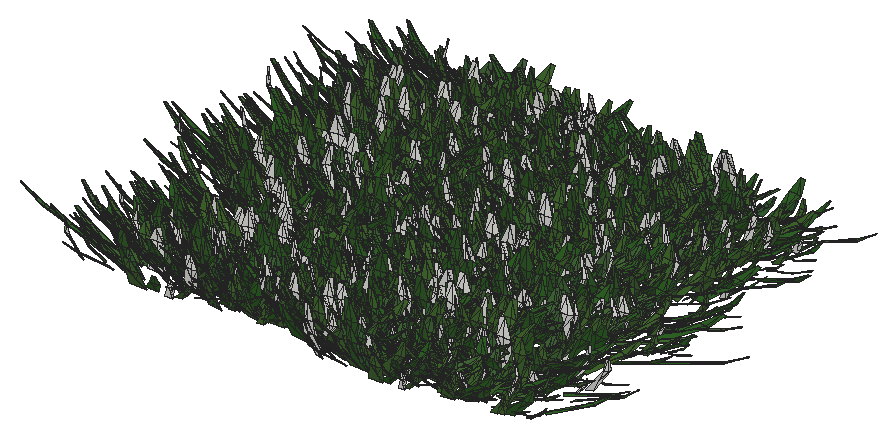
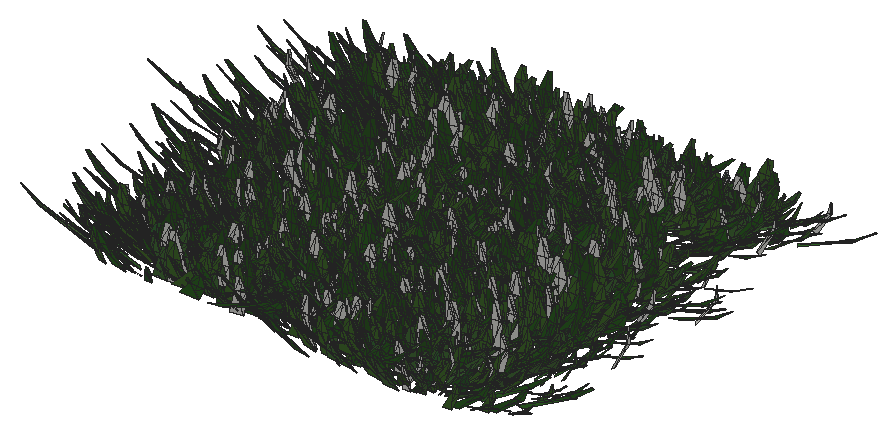
# SketchUp Ruby script. Lengths in inches.
U = 1.inch
M = Sketchup.active_model
def pt(a) = Geom::Point3d.new(a.map { |v| v * U })
def face(e, loops, mat)
  f = e.add_face(loops[0].map { |a| pt(a) })
  loops[1..].each { |l| e.add_face(l.map { |a| pt(a) }).erase! }
  f.material = f.back_material = mat if mat
  f
end
# faces: each face lists its corners as indices into pts; further lists are holes
def faces(e, pts, list, mat = nil) = list.each { |f| face(e, (f[0].is_a?(Array) ? f : [f]).map { |l| l.map { |i| pts[i] } }, mat) }
# xy, xz, yz: faces in a plane at the given z, y or x. An outline is a flat list of corners, or four numbers for a rectangle; further outlines are holes
def ring(l) = l.size == 4 ? [[l[0], l[1]], [l[2], l[1]], [l[2], l[3]], [l[0], l[3]]] : l.each_slice(2).to_a
def flat(e, list, mat, &to3) = list.each { |f| face(e, (f[0].is_a?(Array) ? f : [f]).map { |l| ring(l).map { |u, v| to3.(u, v) } }, mat) }
def xy(e, z, list, mat = nil) = flat(e, list, mat) { |x, y| [x, y, z] }
def xz(e, y, list, mat = nil) = flat(e, list, mat) { |x, z| [x, y, z] }
def yz(e, x, list, mat = nil) = flat(e, list, mat) { |y, z| [x, y, z] }
def lines(e, pts, list) = list.each { |a, b| e.add_line(pt(pts[a]), pt(pts[b])) }
# prism: a flat outline (further loops are holes) pulled along v
def prism(e, loops, v, mat = nil)
  f = face(e, loops, mat); d = Geom::Vector3d.new(v.map { |x| x * U })
  f.pushpull(f.normal.samedirection?(d) ? d.length : -d.length)
end
def box(e, o, s, mat = nil) = prism(e, [[o, [o[0] + s[0], o[1], o[2]], [o[0] + s[0], o[1] + s[1], o[2]], [o[0], o[1] + s[1], o[2]]]], [0, 0, s[2]], mat)
def at(x, y, z, deg = 0) = Geom::Transformation.translation(pt([x, y, z])) * Geom::Transformation.rotation(ORIGIN, Z_AXIS, deg.degrees)
def axes(o, x, y, z) = Geom::Transformation.new([*x, 0, *y, 0, *z, 0, *pt(o).to_a, 1])
def part(name) = M.definitions.add(name)
# library, detail: a bought-in or finely detailed component or shape, given as its bounding box
def library(name, o, s) = part(name).tap { |d| box(d.entities, o, s) }
def detail(e, o, s) = box(e.add_group.entities, o, s)
def put(e, d, t, mat = nil) = e.add_instance(d, t).tap { |i| i.material = mat if mat }
def group(e, t, mat = nil) = e.add_group.tap { |g| g.transformation = t; g.material = mat if mat }.entities
root = M.entities
M.materials.add("Material10").color = [48, 100, 38]
M.materials.add("Material3").color = [68, 110, 58]
M.materials.add("Material4").color = [48, 90, 38]
M.materials.add("Material5").color = [68, 110, 48]
M.materials.add("Material6").color = [48, 90, 48]
M.materials.add("Material7").color = [58, 110, 58]
M.materials.add("Material8").color = [58, 90, 38]
M.materials.add("Material9").color = [68, 100, 58]
c1 = part("grass00")
p = [[-0.6875,0.15,0],[-0.56,0.08,5.52],[-0.04,0.03,2.76],[0.48,-0.02,0],[0.35,-0.02,5.52],[-0.1,-0.14,5.52],
  [-0.12,0.65,8.37],[-0.42,0.65,8.37]]
faces(c1.entities,p,[[0,1,2,3],[3,2,4],[1,5,2],[5,4,2],[1,6,5],[4,5,6],[7,6,1]])
c2 = part("Group16\#1")
put(c2.entities,c1,axes([1.44,-0.61,-0.01],[0.05352,0.12609,0],[-0.10704,0.04543,0.07239],[0.06664,-0.02828,0.11628]),"Material6")
put(c2.entities,c1,axes([0.76,-0.15,-0.01],[0.04676,0.24062,0],[-0.23162,0.04501,0.06642],[0.0652,-0.01267,0.23595]),"Material3")
put(c2.entities,c1,axes([0.79,0.01,-0.01],[-0.00606,0.34651,0],[-0.34381,-0.00602,0.0432],[0.04319,0.00076,0.34386]))
put(c2.entities,c1,axes([1,0.23,-0.01],[-0.07192,0.31144,0],[-0.28722,-0.06632,0.1236],[0.12043,0.02781,0.29478]),"Material5")
put(c2.entities,c1,axes([1.66,0.77,-0.01],[-0.13828,0.29651,0],[-0.21551,-0.1005,0.22471],[0.20365,0.09498,0.23779]),"Material10")
put(c2.entities,c1,axes([0.6875,0.52,-0.01],[-0.18126,0.24051,0],[-0.22746,-0.17142,0.09788],[0.07817,0.05891,0.28481]),"Material5")
put(c2.entities,c1,axes([0.68,0.78,-0.01],[-0.215,0.18688,0],[-0.12385,-0.14248,0.21334],[0.13995,0.16101,0.18878]),"Material3")
put(c2.entities,c1,axes([0.56,1,-0.01],[-0.13756,0.07624,0],[-0.06159,-0.11112,0.0927],[0.04494,0.08108,0.12705]),"Material5")
put(c2.entities,c1,axes([0.2,0.64,-0.01],[-0.23729,0.07254,0],[-0.05711,-0.18681,0.153],[0.04473,0.14632,0.19535]),"Material10")
put(c2.entities,c1,axes([0.0625,0.72,-0.01],[-0.28874,0.02525,0],[-0.02179,-0.24916,0.14647],[0.01276,0.14591,0.25012]),"Material3")
put(c2.entities,c1,axes([-0.08,0.62,-0.01],[-0.34089,-0.04187,0],[0.03255,-0.26504,0.216],[-0.02633,0.21439,0.26703]),"Material10")
put(c2.entities,c1,axes([-0.34,0.98,-0.01],[-0.14314,-0.0493,0],[0.04397,-0.12769,0.06843],[-0.02228,0.0647,0.13505]),"Material10")
put(c2.entities,c1,axes([-0.87,1.45,-0.01],[-0.23488,-0.14114,0],[0.13761,-0.22901,0.06087],[-0.03135,0.05217,0.26717]))
put(c2.entities,c1,axes([-0.72,0.77,-0.01],[-0.14208,-0.13251,0],[0.07209,-0.0773,0.16301],[-0.11118,0.11922,0.1057]),"Material10")
put(c2.entities,c1,axes([-0.62,0.43,-0.01],[-0.14845,-0.21203,0],[0.18654,-0.13061,0.12304],[-0.10079,0.07057,0.22772]),"Material3")
put(c2.entities,c1,axes([-0.68,0.29,-0.01],[-0.13639,-0.32136,0],[0.31723,-0.13464,0.05579],[-0.05136,0.0218,0.34462]),"Material4")
put(c2.entities,c1,axes([-0.64,0.125,-0.01],[-0.0458,-0.23569,0],[0.22124,-0.043,0.08276],[-0.08124,0.01579,0.22538]),"Material7")
put(c2.entities,c1,axes([-1.6,-0.03,-0.01],[0.00576,-0.32897,0],[0.27526,0.00482,0.18018],[-0.18015,-0.00315,0.2753]),"Material5")
put(c2.entities,c1,axes([-1.36,-0.31,-0.01],[0.05718,-0.24765,0],[0.18172,0.04196,0.17267],[-0.16825,-0.03885,0.1865]),"Material10")
put(c2.entities,c1,axes([-1.54,-0.72,-0.01],[0.06537,-0.14017,0],[0.13555,0.06321,0.03939],[-0.0357,-0.01665,0.14956]))
put(c2.entities,c1,axes([-1.19,-0.9,-0.01],[0.09597,-0.12735,0],[0.11214,0.08451,0.07557],[-0.06035,-0.04548,0.14042]),"Material9")
put(c2.entities,c1,axes([-0.47,-0.54,-0.01],[0.11588,-0.10072,0],[0.0618,0.0711,0.12124],[-0.07953,-0.0915,0.0942]))
put(c2.entities,c1,axes([-0.47,-0.84,-0.01],[0.11927,-0.0661,0],[0.06603,0.11913,0.00646],[-0.00313,-0.00565,0.13621]),"Material5")
put(c2.entities,c1,axes([-0.38,-1.24,-0.01],[0.28037,-0.08571,0],[0.0618,0.20215,0.20315],[-0.05939,-0.19428,0.21139]),"Material9")
put(c2.entities,c1,axes([-0.06,-0.66,-0.01],[0.22719,-0.01987,0],[0.01247,0.14255,0.17758],[-0.01547,-0.17691,0.1431]),"Material8")
put(c2.entities,c1,axes([0.11,-0.89,-0.01],[0.14882,0.01828,0],[-0.01058,0.08611,0.12229],[0.01491,-0.12138,0.08676]),"Material6")
put(c2.entities,c1,axes([0.25,-0.72,-0.01],[0.20481,0.07053,0],[-0.06206,0.18022,0.10291],[0.03351,-0.0973,0.1906]),"Material6")
put(c2.entities,c1,axes([0.85,-1.42,-0.01],[0.16481,0.09904,0],[-0.09472,0.15762,0.05616],[0.02893,-0.04814,0.18389]),"Material5")
put(c2.entities,c1,axes([1.01,-1.09,-0.01],[0.21858,0.20385,0],[-0.17495,0.1876,0.15339],[0.10462,-0.11218,0.25652]),"Material10")
put(c2.entities,c1,axes([1.01,-0.71,-0.01],[0.08733,0.12473,0],[-0.06445,0.04512,0.13037],[0.1068,-0.07477,0.07867]),"Material6")
c3 = part("Group15\#1")
put(c3.entities,c2,at(0,0,0))
c4 = part("3darcstudiotree_grass00\#1")
put(c4.entities,c3,at(0,0,0))
put(root,c4,axes([93.18,67.32,7.6],[-0.51089,-1.13336,0],[4.16419,-0.11732,-0.02839],[0.14199,-0.004,1.31807]))
put(root,c4,axes([93.3,71.95,7.6],[-2.45945,-0.81694,0],[3.01218,-0.56677,-0.02546],[0.16778,-0.03157,1.94365]))
put(root,c4,axes([93.95,78.48,7.6],[-3.46196,-0.96436,0],[3.51371,-0.78837,-0.02493],[0.09006,-0.02021,1.43253]))
put(root,c4,axes([93.67,81.3,7.6],[-4.50327,-0.2714,0],[0.9427,-0.97764,-0.01967],[0.02949,-0.03058,1.60841]))
put(root,c4,axes([92.97,60.17,7.6],[-2.75992,0.94196,0],[-2.97534,-0.54485,-0.02032],[-0.11782,-0.02158,1.65635]))
put(root,c4,axes([93.67,46.37,7.6],[-4.30976,0.17306,0],[-0.69895,-1.08789,-0.04907],[-0.04617,-0.07186,1.63442]))
put(root,c4,axes([93.23,73.76,7.6],[1.62415,-0.82572,0],[3.47351,0.42701,-0.04022],[0.29805,0.03664,1.99791]))
put(root,c4,axes([92.31,44.43,7.6],[-0.21475,1.16093,0],[-4.31768,-0.04992,-0.00948],[-0.04784,-0.00055,1.36423]))
put(root,c4,axes([94.23,74.96,7.6],[-1.92009,-1.06648,0],[4.1428,-0.46617,-0.04331],[0.26264,-0.02955,1.88835]))
put(root,c4,axes([94.39,76.8,7.6],[-1.61898,-1.19321,0],[3.76246,-0.31906,-0.01224],[0.0924,-0.00784,1.97883]))
put(root,c4,axes([92.45,61.43,7.6],[0.9763,1.20206,0],[-4.96643,0.2521,-0.02679],[-0.14937,0.00758,1.80175]))
put(root,c4,axes([93.08,47.52,7.6],[3.61009,-0.1138,0],[0.57858,1.14719,-0.05027],[0.03392,0.06725,1.55905]))
put(root,c4,axes([92.44,70.35,7.6],[2.01763,0.79304,0],[-4.00397,0.63667,-0.00074],[-0.00407,0.00065,1.93092]))
put(root,c4,axes([94.01,55.67,7.6],[3.2052,-0.51026,0],[2.09643,0.82305,-0.0345],[0.14052,0.05517,1.8497]))
put(root,c4,axes([94.22,49.64,7.6],[0.11052,0.97112,0],[-4.47276,0.03182,-0.02239],[-0.14712,0.00105,1.83839]))
put(root,c4,axes([94.31,65.74,7.6],[-0.51157,1.00032,0],[-4.92552,-0.15743,-0.0277],[-0.16641,-0.00532,1.87956]))
put(root,c4,axes([96.53,58.84,7.6],[-2.88645,-0.88877,0],[3.86578,-0.78468,-0.02494],[0.12186,-0.02474,1.95866]))
put(root,c4,axes([96.49,82.53,7.6],[-4.37,-0.28374,0],[1.17026,-1.12647,-0.00758],[0.01125,-0.01083,1.7185]))
put(root,c4,axes([96.19,65.93,7.6],[-0.06579,-0.95839,0],[4.48291,-0.01923,-0.0405],[0.2731,-0.00117,1.89003]))
put(root,c4,axes([96.62,70.86,7.6],[-1.52084,-1.07462,0],[3.90834,-0.3457,-0.03351],[0.20602,-0.01822,1.68972]))
put(root,c4,axes([97.3,77.97,7.6],[-1.03944,-1.24074,0],[4.69727,-0.24595,-0.02019],[0.11188,-0.00586,1.69814]))
put(root,c4,axes([97.11,81.66,7.6],[-0.98612,-1.22055,0],[4.4455,-0.22448,-0.03802],[0.23503,-0.01187,1.78771]))
put(root,c4,axes([97.47,60.42,7.6],[-3.13643,-0.44743,0],[1.98712,-0.87059,-0.04344],[0.16835,-0.07376,1.9596]))
put(root,c4,axes([97.73,52.01,7.6],[-1.81933,-1.05694,0],[4.48084,-0.48206,-0.04688],[0.23644,-0.02544,1.67419]))
put(root,c4,axes([97.66,56.53,7.6],[-3.96294,0.68936,0],[-2.37942,-0.85491,-0.01001],[-0.0292,-0.01049,1.32974]))
put(root,c4,axes([98.77,64.52,7.6],[-0.37875,-1.01008,0],[4.48858,-0.10519,-0.00863],[0.04422,-0.00104,1.44957]))
put(root,c4,axes([99.4,55.39,7.6],[-1.70482,-1.13891,0],[4.74643,-0.44405,-0.05081],[0.22443,-0.021,1.49393]))
put(root,c4,axes([97.86,62.77,7.6],[4.79231,-0.42159,0],[1.43855,1.02203,-0.0057],[0.01193,0.00848,1.70987]))
put(root,c4,axes([99.49,75.21,7.6],[-0.51771,-1.03917,0],[4.88499,-0.15211,-0.06365],[0.38906,-0.01211,1.89522]))
put(root,c4,axes([99.04,72.46,7.6],[2.41645,-0.95234,0],[3.1357,0.49728,-0.01781],[0.0973,0.01543,1.50117]))
put(root,c4,axes([98.65,80.14,7.6],[3.95263,-0.39442,0],[1.50714,0.94398,-0.02611],[0.05477,0.0343,1.43783]))
put(root,c4,axes([99.95,47.45,7.6],[-4.30049,-0.11953,0],[0.50316,-1.13147,-0.05312],[0.03445,-0.07747,1.67036]))
put(root,c4,axes([98.75,46.06,7.6],[4.68959,-0.46091,0],[1.44891,0.92138,-0.00849],[0.02258,0.01436,1.79934]))
put(root,c4,axes([100.16,68.92,7.6],[0.57687,-1.07494,0],[3.69634,0.12398,-0.00096],[0.00701,0.00024,1.71349]))
put(root,c4,axes([100.13,67.55,7.6],[-4.14654,0.02565,0],[-0.12263,-1.23885,-0.01248],[-0.00137,-0.01382,1.37214]))
put(root,c4,axes([100.37,76.89,7.6],[-3.83685,0.38096,0],[-1.50034,-0.94442,-0.04199],[-0.1028,-0.06471,1.68502]))
put(root,c4,axes([100.19,61.53,7.6],[-4.14844,0.73182,0],[-2.28116,-0.8082,0],[-0.00002,-0.00001,1.91868]))
put(root,c4,axes([99.38,45.07,7.6],[3.44069,0.27197,0],[-1.2898,1.01983,-0.04459],[-0.0839,0.06634,1.66873]))
put(root,c4,axes([100.69,73.42,7.6],[-4.43528,0.66628,0],[-1.93205,-0.80382,-0.02116],[-0.06942,-0.02888,1.49339]))
put(root,c4,axes([100.37,49.59,7.6],[-2.3482,0.69512,0],[-3.39481,-0.71676,-0.03207],[-0.17565,-0.03709,1.99077]))
put(root,c4,axes([100.57,50.99,7.6],[-3.32313,0.94443,0],[-3.84247,-0.84503,-0.06393],[-0.21081,-0.04636,1.40472]))
put(root,c4,axes([100.375,53.48,7.6],[4.99296,-0.12006,0],[0.49346,1.28259,-0.06081],[0.02614,0.06795,1.44654]))
put(root,c4,axes([102.42,64.07,7.6],[-0.04021,-0.94349,0],[5.12162,-0.01364,-0.05216],[0.22205,-0.00059,1.36288]))
put(root,c4,axes([102.53,53.98,7.6],[0.15214,-1.25594,0],[4.48063,0.03392,-0.01983],[0.10676,0.00081,1.50947]))
put(root,c4,axes([102.81,76.83,7.6],[-0.76774,-1.16095,0],[4.52934,-0.18721,-0.0168],[0.08958,-0.0037,1.55067]))
put(root,c4,axes([102.96,56.75,7.6],[-4.11234,-0.7945,0],[2.93722,-0.95019,-0.06061],[0.1773,-0.05736,1.43628]))
put(root,c4,axes([102.44,65.58,7.6],[-0.59166,-1.13858,0],[3.64186,-0.11828,-0.04034],[0.25705,-0.00835,1.47504]))
put(root,c4,axes([102.7,62.67,7.6],[-3.92438,0.31948,0],[-1.16946,-0.89782,-0.04555],[-0.09619,-0.07385,1.60995]))
put(root,c4,axes([103.21,47.54,7.6],[-4.2338,0.39742,0],[-1.47473,-0.9819,-0.01194],[-0.02743,-0.01826,1.71307]))
put(root,c4,axes([103.43,52.7,7.6],[-3.93577,0.74976,0],[-2.5237,-0.82799,-0.04347],[-0.16838,-0.05524,1.66314]))
put(root,c4,axes([104.29,45.21,7.6],[-3.54943,-0.49503,0],[1.78138,-0.79829,-0.00653],[0.02016,-0.00904,1.4475]))
put(root,c4,axes([104.66,75.52,7.6],[-3.36621,-0.95264,0],[2.81846,-0.62245,-0.00245],[0.01476,-0.00326,1.8862]))
put(root,c4,axes([102.77,79.625,7.6],[0.43598,1.04612,0],[-4.32547,0.11267,-0.02993],[-0.17694,0.00461,1.61572]))
put(root,c4,axes([102.875,61.18,7.6],[-0.51235,0.89086,0],[-4.17612,-0.15011,-0.00494],[-0.0262,-0.00094,1.4129]))
put(root,c4,axes([104.84,49.36,7.6],[0.5765,-1.16396,0],[4.70538,0.14566,-0.00236],[0.01265,0.00039,1.5989]))
put(root,c4,axes([103.43,77.9,7.6],[4.23792,-0.23922,0],[0.87195,0.96546,-0.03599],[0.04234,0.04688,1.32194]))
put(root,c4,axes([104.61,67.62,7.6],[-4.26388,0.42681,0],[-1.64791,-1.02893,-0.00598],[-0.01365,-0.00852,1.70205]))
put(root,c4,axes([103.68,50.48,7.6],[4.67345,-0.08796,0],[0.29357,0.97489,-0.02417],[0.01343,0.0446,1.80918]))
put(root,c4,axes([103.74,80.78,7.6],[0.19862,1.12263,0],[-4.23211,0.0468,-0.03464],[-0.20461,0.00226,1.56527]))
put(root,c4,axes([103.5,82.27,7.6],[2.93954,0.6812,0],[-3.37406,0.90999,-0.0132],[-0.04593,0.01239,1.58767]))
put(root,c4,axes([105.44,58.21,7.6],[-4.4154,0.08876,0],[-0.37121,-1.15413,-0.04274],[-0.0155,-0.04821,1.31001]))
put(root,c4,axes([105.82,68.79,7.6],[-2.79225,-0.78906,0],[3.01148,-0.66605,-0.02762],[0.13842,-0.03061,1.68176]))
put(root,c4,axes([103.9375,59.62,7.6],[2.75191,0.75526,0],[-3.57518,0.81417,-0.05824],[-0.22433,0.05109,1.57486]))
put(root,c4,axes([105.22,71.79,7.6],[2.32702,-1.05964,0],[3.64306,0.50002,-0.02765],[0.14347,0.01969,1.53783]))
put(root,c4,axes([104.48,46.23,7.6],[2.82481,0.56439,0],[-2.40364,0.7519,-0.04441],[-0.20419,0.06387,1.772]))
put(root,c4,axes([105.49,73.35,7.6],[2.47739,-0.8352,0],[3.76427,0.69785,-0.03781],[0.14929,0.02768,1.4396]))
put(root,c4,axes([104.58,70.29,7.6],[0.70904,1.19285,0],[-3.93143,0.14606,-0.03328],[-0.20326,0.00755,1.53387]))
put(root,c4,axes([105.76,55.17,7.6],[1.81143,0.91865,0],[-4.40364,0.5427,-0.01549],[-0.06434,0.00793,1.42146]))
put(root,c4,axes([108.75,45.9,7.6],[-2.19017,-0.8406,0],[3.99666,-0.65083,-0.00487],[0.02392,-0.0039,1.74651]))
put(root,c4,axes([108.51,80.16,7.6],[-4.47501,0.4091,0],[-1.26068,-0.86189,-0.04181],[-0.08597,-0.05877,1.37365]))
put(root,c4,axes([108.81,68.65,7.6],[1.03732,-1.10415,0],[4.61468,0.27096,-0.04288],[0.24016,0.0141,1.70449]))
put(root,c4,axes([109.03,47.83,7.6],[0.84131,-0.93334,0],[4.465,0.25155,-0.02216],[0.11535,0.0065,1.52603]))
put(root,c4,axes([109.72,73.17,7.6],[-4.69083,0.06991,0],[-0.27853,-1.16812,-0.00226],[-0.00086,-0.00362,1.87745]))
put(root,c4,axes([109.36,76.69,7.6],[1.83497,-0.94895,0],[3.86157,0.46669,-0.03335],[0.17925,0.02166,1.60043]))
put(root,c4,axes([110.03,54.01,7.6],[-0.52129,-1.09873,0],[4.55576,-0.13509,-0.02638],[0.13198,-0.00391,1.44452]))
put(root,c4,axes([108.98,70.7,7.6],[4.54978,-0.41024,0],[1.68506,1.16802,-0.06016],[0.10033,0.06955,1.52593]))
put(root,c4,axes([109.26,59.98,7.6],[-1.83035,0.9083,0],[-3.79147,-0.47752,-0.03585],[-0.1914,-0.02411,1.58646]))
put(root,c4,axes([109.91,64.55,7.6],[-3.83368,0.65394,0],[-2.36906,-0.86802,-0.04776],[-0.17139,-0.0628,1.6727]))
put(root,c4,axes([109.2,58.79,7.6],[4.16884,-0.44191,0],[1.67994,0.9905,-0.02583],[0.06325,0.03729,1.68703]))
put(root,c4,axes([109.64,78.27,7.6],[5.02787,-0.3126,0],[0.9305,0.9354,-0.00031],[0.00054,0.00054,1.72722]))
put(root,c4,axes([110.24,54.98,7.6],[3.79189,-0.60703,0],[2.47223,0.9652,-0.00312],[0.00888,0.00347,1.51309]))
put(root,c4,axes([109.83,57.1,7.6],[4.87895,-0.29762,0],[0.96688,0.99066,-0.01844],[0.03122,0.03199,1.82062]))
put(root,c4,axes([110.87,72.01,7.6],[2.31216,-0.81915,0],[3.42555,0.60431,-0.01427],[0.0583,0.01029,1.30992]))
put(root,c4,axes([110.97,50.59,7.6],[2.96673,-0.89554,0],[3.5792,0.74107,-0.01649],[0.07862,0.01628,1.79785]))
put(root,c4,axes([111.77,66.37,7.6],[-2.17941,-0.94456,0],[3.95832,-0.57082,-0.05686],[0.22617,-0.03262,1.31145]))
put(root,c4,axes([111.75,81.08,7.6],[-5.07724,0.11974,0],[-0.34282,-0.90851,-0.02738],[-0.01844,-0.04887,1.63584]))
put(root,c4,axes([111.4,63.1,7.6],[1.32432,-1.09589,0],[4.49114,0.3392,-0.03916],[0.2319,0.01751,1.81408]))
put(root,c4,axes([109.81,67.32,7.6],[2.43888,0.92157,0],[-4.2022,0.69505,-0.02773],[-0.11094,0.01835,1.51065]))
put(root,c4,axes([110.67,75.22,7.6],[0.35474,0.89706,0],[-4.2384,0.10475,-0.01511],[-0.11034,0.00273,1.95375]))
put(root,c4,axes([110.88,48.82,7.6],[3.6065,0.55096,0],[-2.61428,1.06954,-0.04231],[-0.13529,0.05535,1.92144]))
put(root,c4,axes([112.76,52.65,7.6],[-4.74317,0.13037,0],[-0.40737,-0.92635,-0.04038],[-0.03022,-0.06871,1.5952]))
put(root,c4,axes([112.37,44.9,7.6],[-2.66919,0.82783,0],[-2.98072,-0.60068,-0.02131],[-0.13141,-0.02648,1.8955]))
put(root,c4,axes([112.3125,61.81,7.6],[-1.19355,0.89536,0],[-3.41467,-0.28449,-0.02384],[-0.1819,-0.01516,1.80943]))
put(root,c4,axes([114.39,67.45,7.6],[0.34278,-0.91027,0],[3.93669,0.09265,-0.01523],[0.12213,0.00287,1.99019]))
put(root,c4,axes([115,48.82,7.6],[-3.72708,-0.77449,0],[2.33482,-0.70224,-0.01701],[0.09318,-0.02803,1.95649]))
put(root,c4,axes([115.39,57.9375,7.6],[-3.89564,-0.27559,0],[0.99686,-0.8807,-0.03071],[0.05069,-0.04478,1.38702]))
put(root,c4,axes([114.85,54.25,7.6],[1.68583,-0.81683,0],[4.11916,0.53134,-0.04957],[0.26252,0.03386,1.72633]))
put(root,c4,axes([115.37,75.38,7.6],[-0.13589,-1.00462,0],[3.6498,-0.03085,-0.02047],[0.14931,-0.00126,1.66543]))
put(root,c4,axes([115.07,52.55,7.6],[2.09408,-1.17299,0],[4.38498,0.48927,-0.04062],[0.22124,0.02469,1.79015]))
put(root,c4,axes([114.99,73.53,7.6],[-3.01773,0.80944,0],[-3.41595,-0.79595,-0.00031],[-0.00127,-0.0003,1.61707]))
put(root,c4,axes([114.92,57.27,7.6],[3.44538,-0.3202,0],[1.49096,1.00268,-0.02775],[0.06957,0.04678,1.92398]))
put(root,c4,axes([115.21,43.84,7.6],[-1.08515,0.9046,0],[-3.54235,-0.26559,-0.04553],[-0.24621,-0.01846,1.30482]))
put(root,c4,axes([116.45,63.28,7.6],[-0.65047,-1.04109,0],[4.03064,-0.1574,-0.04759],[0.24886,-0.00972,1.34947]))
put(root,c4,axes([117.06,72.16,7.6],[-2.08423,-0.85727,0],[3.21957,-0.48922,-0.04312],[0.30054,-0.04567,1.92045]))
put(root,c4,axes([117.25,78.55,7.6],[-2.32935,-0.7629,0],[3.09102,-0.58986,-0.04177],[0.18704,-0.03569,1.36919]))
put(root,c4,axes([117.375,55.34,7.6],[1.57863,-1.11612,0],[3.5477,0.31361,-0.02361],[0.12493,0.01104,1.32009]))
put(root,c4,axes([116.32,76.9375,7.6],[1.59781,1.17762,0],[-4.51681,0.38303,-0.04327],[-0.24194,0.02052,1.7601]))
put(root,c4,axes([116.54,68.84,7.6],[0.44983,1.23092,0],[-3.94694,0.09015,-0.02215],[-0.12679,0.0029,1.42375]))
put(root,c4,axes([117.83,71.05,7.6],[1.0564,-1.26283,0],[3.63785,0.1902,-0.01603],[0.10027,0.00524,1.48463]))
put(root,c4,axes([116.75,51.42,7.6],[-0.94273,1.27464,0],[-5.04874,-0.23338,-0.00297],[-0.01721,-0.0008,1.8915]))
put(root,c4,axes([117.08,80.68,7.6],[4.33399,-0.08203,0],[0.31572,1.04255,-0.04662],[0.02263,0.07473,1.68074]))
put(root,c4,axes([117.24,80.11,7.6],[-0.71459,1.01896,0],[-4.19391,-0.18382,-0.02601],[-0.15992,-0.00701,1.66111]))
put(root,c4,axes([116.67,46.3125,7.6],[3.19575,0.75582,0],[-3.09164,0.817,-0.00432],[-0.01514,0.004,1.43292]))
put(root,c4,axes([118.05,65.93,7.6],[3.81417,-0.56994,0],[2.46568,1.03131,-0.05659],[0.15929,0.06663,1.64805]))
put(root,c4,axes([117.45,44.72,7.6],[4.81538,0.36393,0],[-1.10544,0.91418,-0.04581],[-0.0874,0.07228,1.57403]))
put(root,c4,axes([117.42,64.66,7.6],[3.74971,0.70366,0],[-2.74434,0.91401,-0.02233],[-0.09238,0.03077,1.9689]))
put(root,c4,axes([118.21,60.08,7.6],[-2.89172,1.0734,0],[-3.89316,-0.6555,-0.0002],[-0.00109,-0.00018,1.96126]))
put(root,c4,axes([118.58,61.02,7.6],[4.74483,-0.24076,0],[0.85247,1.04999,-0.04034],[0.05471,0.06739,1.82611]))
put(root,c4,axes([120.57,78.18,7.6],[-3.63628,-0.62096,0],[2.92947,-1.07217,-0.03279],[0.09663,-0.03537,1.69581]))
put(root,c4,axes([118.55,48.375,7.6],[4.00198,0.55005,0],[-2.10991,0.95943,-0.0244],[-0.05644,0.02566,1.31386]))
put(root,c4,axes([121.19,61.59,7.6],[-4.89778,-0.29998,0],[1.23144,-1.25658,-0.038],[0.05293,-0.05401,1.89315]))
put(root,c4,axes([121.16,73.79,7.6],[3.74508,0.15378,0],[-0.63868,0.9721,-0.00501],[-0.00465,0.00708,1.40942]))
put(root,c4,axes([121.09,80.23,7.6],[0.68514,1.26478,0],[-4.89254,0.16565,-0.03426],[-0.19489,0.0066,1.77113]))
put(root,c4,axes([121.86,69.22,7.6],[3.3533,-0.38731,0],[1.56438,0.84651,-0.0238],[0.08194,0.04434,1.9133]))
put(root,c4,axes([122.375,56.97,7.6],[2.65179,-0.82671,0],[3.59664,0.72105,-0.04277],[0.18565,0.03722,1.60323]))
put(root,c4,axes([123.43,49.51,7.6],[-4.93357,-0.09351,0],[0.37181,-1.22601,-0.05601],[0.01916,-0.06319,1.39118]))
put(root,c4,axes([123.57,52.4,7.6],[-3.34759,-0.83293,0],[3.286,-0.82541,-0.05331],[0.22185,-0.05573,1.71744]))
put(root,c4,axes([123.56,50.52,7.6],[0.64604,-1.03899,0],[4.47986,0.1741,-0.01704],[0.10727,0.00417,1.80481]))
put(root,c4,axes([121.97,47.5,7.6],[1.02925,1.26191,0],[-4.50486,0.22964,-0.03996],[-0.19294,0.00984,1.416]))
put(root,c4,axes([121.98,67.21,7.6],[2.0369,1.16411,0],[-3.53478,0.38656,-0.02724],[-0.15553,0.01701,1.50258]))
put(root,c4,axes([122.29,55.86,7.6],[4.16551,0.00829,0],[-0.03133,0.98341,-0.01492],[-0.00089,0.02794,1.84219]))
put(root,c4,axes([122.33,45,7.6],[3.29102,0.44295,0],[-1.77478,0.82413,-0.02125],[-0.05688,0.02641,1.32121]))
put(root,c4,axes([123.28,80.73,7.6],[-2.38266,1.15159,0],[-4.35256,-0.56285,-0.04288],[-0.20993,-0.02715,1.68813]))
put(root,c4,axes([123.46,62.89,7.6],[-2.09957,0.91209,0],[-4.41964,-0.63586,-0.03664],[-0.13193,-0.01898,1.3241]))
put(root,c4,axes([123.1875,72.28,7.6],[3.03097,0.54961,0],[-2.11734,0.72979,-0.02439],[-0.10216,0.03521,1.60766]))
put(root,c4,axes([123.72,58.375,7.6],[4.80677,-0.31921,0],[1.29296,1.21686,-0.06211],[0.08115,0.07638,1.60192]))
put(root,c4,axes([124.56,75.24,7.6],[1.96449,-0.88015,0],[3.48703,0.48644,-0.05199],[0.25829,0.03603,1.41973]))
put(root,c4,axes([124.22,70.76,7.6],[-2.15894,0.75531,0],[-3.65102,-0.65224,-0.01309],[-0.05957,-0.01064,1.56859]))
put(root,c4,axes([123.46,77.19,7.6],[3.46841,0.85303,0],[-2.60309,0.66151,-0.00671],[-0.03109,0.0079,1.53359]))
put(root,c4,axes([123.43,66.61,7.6],[4.28051,0.69294,0],[-2.55654,0.98703,-0.02279],[-0.07934,0.03063,1.88252]))
put(root,c4,axes([124.06,59.86,7.6],[4.57656,0.58892,0],[-2.21831,1.07741,-0.04224],[-0.10111,0.04911,1.58426]))
put(root,c4,axes([124.51,45.8125,7.6],[3.90944,0.05539,0],[-0.24036,1.06035,-0.02759],[-0.00929,0.04097,1.57942]))
